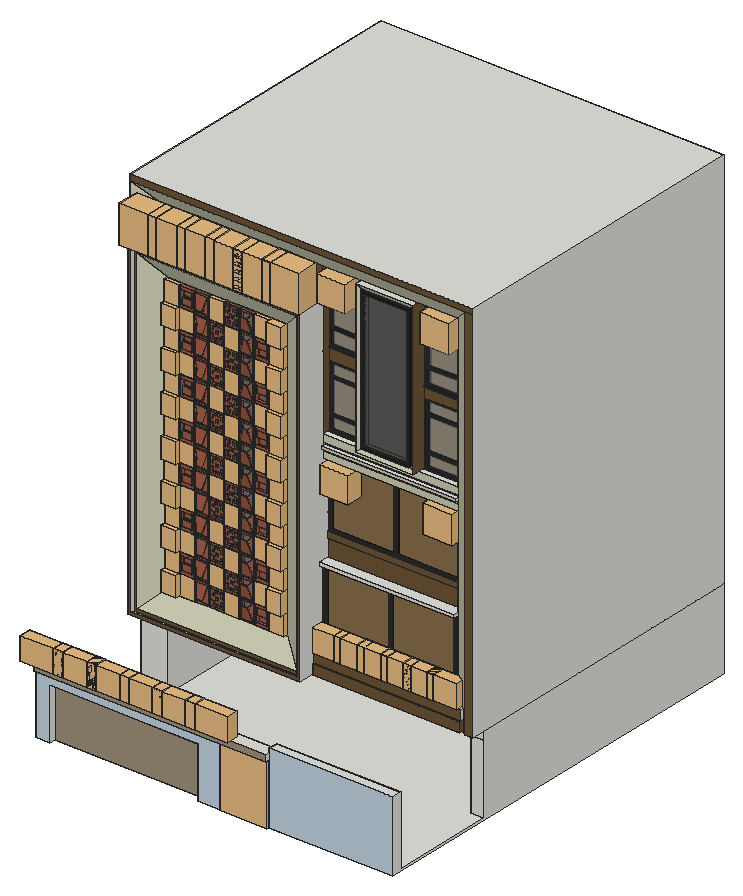
# SketchUp Ruby script. Lengths in inches.
U = 1.inch
M = Sketchup.active_model
def pt(a) = Geom::Point3d.new(a.map { |v| v * U })
def face(e, loops, mat)
  f = e.add_face(loops[0].map { |a| pt(a) })
  loops[1..].each { |l| e.add_face(l.map { |a| pt(a) }).erase! }
  f.material = f.back_material = mat if mat
  f
end
# faces: each face lists its corners as indices into pts; further lists are holes
def faces(e, pts, list, mat = nil) = list.each { |f| face(e, (f[0].is_a?(Array) ? f : [f]).map { |l| l.map { |i| pts[i] } }, mat) }
# xy, xz, yz: faces in a plane at the given z, y or x. An outline is a flat list of corners, or four numbers for a rectangle; further outlines are holes
def ring(l) = l.size == 4 ? [[l[0], l[1]], [l[2], l[1]], [l[2], l[3]], [l[0], l[3]]] : l.each_slice(2).to_a
def flat(e, list, mat, &to3) = list.each { |f| face(e, (f[0].is_a?(Array) ? f : [f]).map { |l| ring(l).map { |u, v| to3.(u, v) } }, mat) }
def xy(e, z, list, mat = nil) = flat(e, list, mat) { |x, y| [x, y, z] }
def xz(e, y, list, mat = nil) = flat(e, list, mat) { |x, z| [x, y, z] }
def yz(e, x, list, mat = nil) = flat(e, list, mat) { |y, z| [x, y, z] }
def lines(e, pts, list) = list.each { |a, b| e.add_line(pt(pts[a]), pt(pts[b])) }
# prism: a flat outline (further loops are holes) pulled along v
def prism(e, loops, v, mat = nil)
  f = face(e, loops, mat); d = Geom::Vector3d.new(v.map { |x| x * U })
  f.pushpull(f.normal.samedirection?(d) ? d.length : -d.length)
end
def box(e, o, s, mat = nil) = prism(e, [[o, [o[0] + s[0], o[1], o[2]], [o[0] + s[0], o[1] + s[1], o[2]], [o[0], o[1] + s[1], o[2]]]], [0, 0, s[2]], mat)
def at(x, y, z, deg = 0) = Geom::Transformation.translation(pt([x, y, z])) * Geom::Transformation.rotation(ORIGIN, Z_AXIS, deg.degrees)
def axes(o, x, y, z) = Geom::Transformation.new([*x, 0, *y, 0, *z, 0, *pt(o).to_a, 1])
def part(name) = M.definitions.add(name)
# library, detail: a bought-in or finely detailed component or shape, given as its bounding box
def library(name, o, s) = part(name).tap { |d| box(d.entities, o, s) }
def detail(e, o, s) = box(e.add_group.entities, o, s)
def put(e, d, t, mat = nil) = e.add_instance(d, t).tap { |i| i.material = mat if mat }
def group(e, t, mat = nil) = e.add_group.tap { |g| g.transformation = t; g.material = mat if mat }.entities
root = M.entities
M.materials.add("Concrete block").color = [182, 184, 178]
M.materials.add("Generic").color = [208, 207, 183]
M.materials.add("Glass_Tinted_Gray").color = [0, 0, 0]
M.materials["Glass_Tinted_Gray"].alpha = 0.125
M.materials.add("Sandstone 150cm").color = [161, 146, 124]
M.materials.add("Walnut Highgloss 300cm").color = [111, 85, 55]
M.materials.add("[0128_White]").color = [255, 255, 255]
M.materials.add("[0135_DarkGray]").color = [81, 81, 81]
M.materials.add("[Color C07]1").color = [160, 91, 69]
M.materials.add("[Color M01]").color = [226, 226, 226]
M.materials.add("[Color M07]").color = [114, 114, 114]
M.materials.add("[Color M08]").color = [30, 30, 30]
M.materials.add("[Granite Dark Gray]").color = [69, 68, 68]
M.materials.add("[Mirror 02]").color = [229, 229, 229]
M.materials.add("[Terrazzo Light Blue]").color = [196, 214, 227]
M.materials.add("[Translucent Glass Gray]").color = [51, 51, 51]
M.materials["[Translucent Glass Gray]"].alpha = 0.78
M.materials.add("[Translucent Glass Gray]2").color = [128, 128, 128]
M.materials["[Translucent Glass Gray]2"].alpha = 0.5
c1 = library("Paired curtain panels",[0.83,0,0],[155.09,8.12,139.81])
c2 = part("PENTEK_RP Fineline 50S_Sliding_DoorCase_E1")
box(c2.entities,[0,0,0],[1.51,3.66,99.27],"[0135_DarkGray]")
c3 = part("PENTEK_RP Fineline 50S_SlidingDooe_Case_E2")
box(c3.entities,[0,0,0],[96.25,3.66,1.51],"[0135_DarkGray]")
c4 = part("pentek_RP Fineline 50S_SlidingDoor_Case")
put(c4.entities,c2,at(97.76,0,0))
put(c4.entities,c3,at(1.51,0,0))
put(c4.entities,c2,at(0,0,0))
put(c4.entities,c3,at(1.51,0,97.76))
c5 = part("PENTEK_RP Fineline 50S_SlidingDoor_GlazingBead_2")
box(c5.entities,[0,0,0],[0.56,0.59,94.39],"[0135_DarkGray]")
c6 = part("PENTEK_RP Fineline 50S_SlidingDoor_Glass")
box(c6.entities,[0,0,0],[46.58,0.16,94.39],"Glass_Tinted_Gray")
c7 = part("PENTEK_RP Fineline 50S_SlidingDoor_GlazingBead")
box(c7.entities,[0,0,0],[45.47,0.59,0.56],"[0135_DarkGray]")
c8 = part("PENTEK_RP Fineline 50S_SlidingDoor_Leaf_E1")
xy(c8.entities,0,[[0,0,0.93,1.97],[0.93,1.57,1.49,1.97]],"[0135_DarkGray]")
xy(c8.entities,96.25,[[0,0,0.93,0,0.93,1.57,1.49,1.57,1.49,1.97,0,1.97]],"[0135_DarkGray]")
xz(c8.entities,0,[[0,0,0.93,96.25]],"[0135_DarkGray]")
xz(c8.entities,1.57,[[0.93,0,1.49,95.32],[0.93,95.32,1.49,96.25]],"[0135_DarkGray]")
xz(c8.entities,1.97,[[0,0,1.49,96.25]],"[0135_DarkGray]")
yz(c8.entities,0,[[0,0,1.97,96.25]],"[0135_DarkGray]")
yz(c8.entities,0.93,[[0,0,1.57,0.93],[0,0.93,1.57,95.32],[0,95.32,1.57,96.25]],"[0135_DarkGray]")
yz(c8.entities,1.49,[[1.57,0,1.97,95.32],[1.57,95.32,1.97,96.25]],"[0135_DarkGray]")
c9 = part("PENTEK_RP Fineline 50S_SlidingDoor_Leaf_E2")
xy(c9.entities,0,[[0,0,0,1.57,0.56,1.57,0.56,1.97,46.02,1.97,46.02,1.57,46.58,1.57,46.58,0]],"[0135_DarkGray]")
xy(c9.entities,0.93,[[0,0,46.58,1.57]],"[0135_DarkGray]")
xy(c9.entities,1.49,[[0.56,1.57,46.02,1.97]],"[0135_DarkGray]")
xz(c9.entities,0,[[0,0,46.58,0.93]],"[0135_DarkGray]")
xz(c9.entities,1.57,[[0,0,0.56,0.93],[46.02,0,46.58,0.93],[0.56,0.93,46.02,1.49]],"[0135_DarkGray]")
xz(c9.entities,1.97,[[0.56,0,46.02,1.49]],"[0135_DarkGray]")
yz(c9.entities,0,[[0,0,1.57,0.93]],"[0135_DarkGray]")
yz(c9.entities,0.56,[[1.57,0,1.97,0.93],[1.57,0.93,1.97,1.49]],"[0135_DarkGray]")
yz(c9.entities,46.02,[[1.57,0,1.97,0.93],[1.57,0.93,1.97,1.49]],"[0135_DarkGray]")
yz(c9.entities,46.58,[[0,0,1.57,0.93]],"[0135_DarkGray]")
c10 = part("PENTEK_RP Fineline S_SlidingDoor_Leaf1")
put(c10.entities,c5,at(0.93,0,0.93))
put(c10.entities,c5,at(46.96,0,0.93))
put(c10.entities,c6,at(1.49,1.42,0.93))
put(c10.entities,c7,at(1.49,0,0.93))
put(c10.entities,c6,at(1.49,0.59,0.93),"[Terrazzo Light Blue]")
put(c10.entities,c8,at(0,0,0))
put(c10.entities,c8,axes([48.44,0,0],[-1,0,0],[0,1,0],[0,0,1]))
put(c10.entities,c9,axes([0.93,0,96.25],[1,0,0],[0,1,0],[0,0,-1]))
put(c10.entities,c9,at(0.93,0,0))
put(c10.entities,c7,at(1.49,0,94.77))
c11 = part("PENTEK_RP Fineline 50S_SlidingDoor_Leaf2")
put(c11.entities,c6,at(1.49,1.42,0.93))
put(c11.entities,c7,at(1.49,0,94.77))
put(c11.entities,c5,at(46.96,0,0.93))
put(c11.entities,c6,at(1.49,0.59,0.93),"[Mirror 02]")
put(c11.entities,c5,at(0.93,0,0.93))
put(c11.entities,c8,at(0,0,0))
put(c11.entities,c8,axes([48.44,0,0],[-1,0,0],[0,1,0],[0,0,1]))
put(c11.entities,c7,at(1.49,0,0.93))
put(c11.entities,c9,axes([0.93,0,96.25],[1,0,0],[0,1,0],[0,0,-1]))
put(c11.entities,c9,at(0.93,0,0))
c12 = part("PENTEK - Slimmest Steel Sliding Door / Window\#1")
put(c12.entities,c4,at(0,-1.88,-0.09))
put(c12.entities,c10,at(1.51,-2.27,1.42))
put(c12.entities,c11,at(49.32,-0.3,1.42))
c13 = part("Agrupar\#57")
prism(c13.entities,[[[1.18,24.41,51.97],[1.18,0,51.97],[1.18,0,0],[1.18,24.41,0]],[[1.18,1.57,50.39],[1.18,22.83,50.39],[1.18,22.83,1.57],[1.18,1.57,1.57]]],[-1.18,0,0])
c14 = part("Agrupar\#59")
box(c14.entities,[0,0,0],[0.24,21.26,16.54])
c15 = part("Agrupar\#58")
prism(c15.entities,[[[0,0,0],[0,0,19.69],[0,24.41,19.69],[0,24.41,0]],[[0,1.57,1.57],[0,22.83,1.57],[0,22.83,18.11],[0,1.57,18.11]]],[1.18,0,0])
c16 = part("Agrupar\#56")
box(c16.entities,[0,0,0],[4.72,24.41,1.57])
c17 = part("Agrupar\#55")
prism(c17.entities,[[[0,0,0],[0,0,97.64],[0,27.56,97.64],[0,27.56,0]],[[0,25.98,1.57],[0,25.98,96.0625],[0,1.57,96.0625],[0,1.57,1.57]]],[4.72,0,0])
c18 = part("Agrupar\#60")
box(c18.entities,[0,0,0],[0.24,21.26,48.82])
c19 = part("Janela Maxim ar")
put(c19.entities,c13,at(1.77,1.57,22.83))
put(c19.entities,c14,at(2.36,3.15,77.95),"[Translucent Glass Gray]2")
put(c19.entities,c15,at(1.77,1.57,1.57))
put(c19.entities,c16,at(0,1.57,74.8))
put(c19.entities,c16,at(0,1.57,21.26))
put(c19.entities,c15,at(1.77,1.57,76.38))
put(c19.entities,c17,at(0,0,0))
put(c19.entities,c14,at(2.36,3.15,3.15),"[Translucent Glass Gray]2")
put(c19.entities,c18,at(2.36,3.15,24.41),"[Translucent Glass Gray]2")
c20 = part("Agrupar\#54")
box(c20.entities,[0,0,0],[7.09,27.56,0.79])
c21 = part("JA-70x250")
put(c21.entities,c19,at(2.36,0,0.79),"[Color M08]")
put(c21.entities,c20,at(0,0,0),"[Granite Dark Gray]")
c22 = library("170_fin_black (1)",[-4.89,-2.76,-3.35],[51.16,5.67,71.46])
c23 = library("Plante \#58",[-0.43,-1.58,0],[20.84,18.06,17.59])
c24 = part("Group\#116")
box(c24.entities,[0,0,0],[5.51,2.76,0.51])
c25 = part("Decorative screen block \#3")
g1 = group(c25.entities,at(0,0,0))
xy(g1,0,[[[0.2,0.2,7.68,7.68],[1.18,1.18,6.69,6.69]]])
xy(g1,0.2,[[[0,0,7.875,7.875],[0.2,0.2,7.68,7.68]]])
xy(g1,3.74,[[[0,0,7.875,7.875],[0.2,0.2,7.68,7.68]]])
xy(g1,3.9375,[[[0.2,0.2,7.68,7.68],[1.18,1.18,6.69,6.69]]])
xz(g1,0,[[0,0.2,7.875,3.74]])
xz(g1,0.2,[[0.2,0,7.68,0.2],[0.2,3.74,7.68,3.9375]])
xz(g1,1.18,[[1.18,0,6.69,3.9375]])
xz(g1,6.69,[[1.18,0,6.69,3.9375]])
xz(g1,7.68,[[0.2,0,7.68,0.2],[0.2,3.74,7.68,3.9375]])
xz(g1,7.875,[[0,0.2,7.875,3.74]])
yz(g1,0,[[0,0.2,7.875,3.74]])
yz(g1,0.2,[[0.2,0,7.68,0.2],[0.2,3.74,7.68,3.9375]])
yz(g1,1.18,[[1.18,0,6.69,3.9375]])
yz(g1,6.69,[[1.18,0,6.69,3.9375]])
yz(g1,7.68,[[0.2,0,7.68,0.2],[0.2,3.74,7.68,3.9375]])
yz(g1,7.875,[[0,0.2,7.875,3.74]])
put(c25.entities,c24,at(1.18,1.18,2.83))
put(c25.entities,c24,at(1.18,3.9375,0.59))
c26 = part("Component\#2")
xy(c26.entities,0,[[[0,0,5.91,5.91],[0.39,0.39,5.51,5.51]]])
xy(c26.entities,2.36,[[[0,0,5.91,5.91],[0.39,0.39,5.51,5.51]],[5.43,5.16,5.51,5.17,5.51,5.51]])
xz(c26.entities,0,[[0,0,5.91,2.36]])
xz(c26.entities,0.39,[[0.39,0,5.51,2.36]])
xz(c26.entities,5.51,[[0.39,0,5.51,2.36]])
xz(c26.entities,5.91,[[0,0,5.91,2.36]])
yz(c26.entities,0,[[0,0,5.91,2.36]])
yz(c26.entities,0.39,[[0.39,0,5.51,0,5.51,2.36,5.23,2.21,0.67,2.21,0.39,2.36],[0.67,2.21,5.23,2.21,5.51,2.36,0.39,2.36]])
yz(c26.entities,4.33,[[1.78,4.3,1.5,4.45,4.41,4.45,4.13,4.3]])
yz(c26.entities,5.51,[[0.39,0,5.17,2.36],[5.17,0,5.51,2.36]])
yz(c26.entities,5.91,[[0,0,5.91,2.36]])
p = [[0.39,0.39,2.36],[4.33,1.5,4.45],[4.33,1.78,4.3],[0.39,0.67,2.21],[5.51,0.39,2.36],[5.51,0.67,2.21],
  [5.43,0.75,2.36],[4.41,1.7,4.16],[0.39,5.23,2.21],[4.33,4.13,4.3],[5.51,5.23,2.21],[5.43,5.16,2.36],
  [4.33,4.41,4.45],[0.39,5.51,2.36],[5.51,5.51,2.36],[5.36,0.89,2.64],[4.49,1.7,4.18],[4.49,4.2,4.18],
  [5.36,5.02,2.64],[5.51,5.17,2.36],[5.51,0.74,2.36]]
faces(c26.entities,p,[[0,1,2,3],[4,0,3,5],[1,4,5,6,7,2],[5,3,2,7,6],[8,10,11,9],[12,13,8,9],[13,14,10,8],[0,4,1],
  [1,12,13,0],[15,16,17,18,19,14,12,1,4,20],[7,16,15,20,6],[9,11,14,12],[14,13,12]])
faces(c26.entities,p,[[8,3,2,9]],"[0128_White]")
c27 = part("Decorative screen block \#2")
xy(c27.entities,0,[[[0.2,0.2,7.68,7.68],[0.82,4.56,2.07,4.56,2.07,5.81,3.3125,5.81,3.3125,7.05,0.82,7.05],[0.82,0.82,3.3125,0.82,3.3125,2.07,2.07,2.07,2.07,3.3125,0.82,3.3125],[4.56,0.82,7.05,0.82,7.05,3.3125,5.81,3.3125,5.81,2.07,4.56,2.07],[5.81,4.56,7.05,4.56,7.05,7.05,4.56,7.05,4.56,5.81,5.81,5.81],[3.3125,3.3125,4.56,4.56]]])
xy(c27.entities,0.2,[[[0,0,7.875,7.875],[0.2,0.2,7.68,7.68]]])
xy(c27.entities,3.74,[[[0,0,7.875,7.875],[0.2,0.2,7.68,7.68]]])
xy(c27.entities,3.9375,[[[0.2,0.2,7.68,7.68],[0.82,0.82,0.82,3.3125,2.07,3.3125,2.07,2.07,3.3125,2.07,3.3125,0.82],[0.82,4.56,0.82,7.05,3.3125,7.05,3.3125,5.81,2.07,5.81,2.07,4.56],[4.56,0.82,4.56,2.07,5.81,2.07,5.81,3.3125,7.05,3.3125,7.05,0.82],[5.81,4.56,5.81,5.81,4.56,5.81,4.56,7.05,7.05,7.05,7.05,4.56],[3.3125,3.3125,4.56,4.56]]])
xz(c27.entities,0,[[0,0.2,7.875,3.74]])
xz(c27.entities,0.2,[[0.2,0,7.68,0.2],[0.2,3.74,7.68,3.9375]])
xz(c27.entities,0.82,[[0.82,0,3.3125,3.9375],[4.56,0,7.05,3.9375]])
xz(c27.entities,2.07,[[2.07,0,3.3125,3.9375],[4.56,0,5.81,3.9375]])
xz(c27.entities,3.3125,[[0.82,0,2.07,3.9375],[3.3125,0,4.56,3.9375],[5.81,0,7.05,3.9375]])
xz(c27.entities,4.56,[[0.82,0,2.07,3.9375],[3.3125,0,4.56,3.9375],[5.81,0,7.05,3.9375]])
xz(c27.entities,5.81,[[2.07,0,3.3125,3.9375],[4.56,0,5.81,3.9375]])
xz(c27.entities,7.05,[[0.82,0,3.3125,3.9375],[4.56,0,7.05,3.9375]])
xz(c27.entities,7.68,[[0.2,0,7.68,0.2],[0.2,3.74,7.68,3.9375]])
xz(c27.entities,7.875,[[0,0.2,7.875,3.74]])
yz(c27.entities,0,[[0,0.2,7.875,3.74]])
yz(c27.entities,0.2,[[0.2,0,7.68,0.2],[0.2,3.74,7.68,3.9375]])
yz(c27.entities,0.82,[[0.82,0,3.3125,3.9375],[4.56,0,7.05,3.9375]])
yz(c27.entities,2.07,[[2.07,0,3.3125,3.9375],[4.56,0,5.81,3.9375]])
yz(c27.entities,3.3125,[[0.82,0,2.07,3.9375],[3.3125,0,4.56,3.9375],[5.81,0,7.05,3.9375]])
yz(c27.entities,4.56,[[0.82,0,2.07,3.9375],[3.3125,0,4.56,3.9375],[5.81,0,7.05,3.9375]])
yz(c27.entities,5.81,[[2.07,0,3.3125,3.9375],[4.56,0,5.81,3.9375]])
yz(c27.entities,7.05,[[0.82,0,3.3125,3.9375],[4.56,0,7.05,3.9375]])
yz(c27.entities,7.68,[[0.2,0,7.68,0.2],[0.2,3.74,7.68,3.9375]])
yz(c27.entities,7.875,[[0,0.2,7.875,3.74]])
c28 = library("Circular opening block",[0,0,-3.9375],[7.875,7.875,7.875])
c29 = library("Decorative screen block \#1",[0,0,0],[7.875,7.875,3.9375])
c30 = library("Decorative screen block",[0,0,0],[7.875,7.875,3.9375])
c31 = library("Group\#2",[0,0,0],[7.875,2.95,7.875])
c32 = library("Group\#18",[0,0,0],[56.8,25.91,35.15])
c33 = part("Group\#19")
put(c33.entities,c32,at(0,0,0))
put(c33.entities,c32,at(88.8,0,0))
put(c33.entities,c32,at(133.08,0,0))
put(c33.entities,c32,at(176.53,0,0))
put(c33.entities,c32,at(44.08,0,0))
put(c33.entities,c32,at(220.58,0,0))
xy(root,-176,[[0,5.8125,0,29.26,29.875,29.26,29.875,909.1875,776.9375,909.1875,776.9375,8.9375,506.3125,8.9375,506.3125,29.26,402.62,29.26,402.62,5.8125,353.78,5.8125,353.78,20,29.875,20,29.875,5.8125]])
xy(root,-169.65,[[29.875,29.26,776.9375,29.26,776.9375,254.75,748.71,254.75,748.71,599.49,87.84,599.49,87.84,254.75,29.875,254.75]])
xy(root,-63.625,[[29.875,5.8125,353.78,20]],"[Color M01]")
xy(root,-42.84,[[0,0,402.62,5.8125],[402.62,0,506.3125,29.26]])
xy(root,-30.4,[[0,0,506.3125,29.26]])
xy(root,-20.71,[[506.3125,8.9375,776.9375,29.26]])
xy(root,-18.41,[[87.84,254.75,748.25,599.49]])
xy(root,0,[[51.21,193.0625,51.21,241.21,69.25,254.75,426.53,254.75,426.53,193.0625],[29.875,225.1875,29.875,254.75,51.21,254.75,51.21,241.21],[428.22,225.1875,428.22,254.75,720.57,254.75,748.19,234.01,748.19,225.1875],[759.9375,225.1875,748.19,234.01,748.19,254.75,776.9375,254.75,776.9375,225.1875],[748.19,234.01,720.57,254.75,748.19,254.75],
  [51.21,241.21,51.21,254.75,69.25,254.75]])
xy(root,6.33,[[57.32,193.0625,418.71,200.1875]])
xy(root,21.47,[[428.22,225.1875,748.19,227.875],[417.03,227.875,428.22,254.75]])
xy(root,42.94,[[417.03,227.875,748.19,227.875,748.19,254.75,720.57,254.75,720.57,396.1875,426.53,396.1875,426.53,254.75,417.03,254.75],[69.25,254.75,337.16,340]])
xy(root,205.02,[[426.53,244,720.57,396.1875]])
xy(root,211.66,[[426.53,244,720.57,268.6875]])
xy(root,250.25,[[426.53,265.8125,720.57,268.6875]],"Walnut Highgloss 300cm")
xy(root,262.7,[[426.53,265.8125,720.57,396.1875]])
xy(root,409.9,[[426.53,254.75,720.57,396.1875]])
xy(root,423.97,[[426.53,254.75,720.57,260.875]])
xy(root,429.89,[[426.53,249.6875,720.57,260.875]])
xy(root,435.28,[[426.53,249.6875,720.57,260.875]])
xy(root,441.875,[[426.53,254.75,720.57,260.875]])
xy(root,456.91,[[509.22,240.4375,635.07,254.75],[426.53,254.75,509.22,301.0625],[635.07,254.75,720.57,328.8125]])
xy(root,472.53,[[524.84,246.3125,619.45,255.3125]])
xy(root,593.92,[[426.53,270.5,509.22,301.0625],[635.07,270.5,720.57,328.8125]],"Walnut Highgloss 300cm")
xy(root,621.56,[[426.53,270.5,720.57,270.5,720.57,332.375,635.07,332.375,635.07,280.1875,509.22,280.1875,509.22,359.25,426.53,359.25]])
xy(root,715.08,[[57.32,193.0625,418.71,200.1875]])
xy(root,723.83,[[51.21,193.0625,426.53,254.75]])
xy(root,770.64,[[524.84,246.3125,619.45,255.3125]])
xy(root,786.25,[[509.22,240.4375,635.07,254.75],[509.22,254.75,635.07,280.1875]])
xy(root,786.25,[[69.25,254.75,337.16,340],[426.53,254.75,509.22,359.25],[635.07,254.75,720.57,332.375]],"Walnut Highgloss 300cm")
xy(root,838.25,[[29.875,225.1875,776.9375,909.1875]])
xz(root,0,[[0,-42.84,506.3125,-30.4]],"Sandstone 150cm")
xz(root,5.8125,[[0,-176,29.875,-176,29.875,-63.625,353.78,-63.625,353.78,-176,402.62,-176,402.62,-42.84,0,-42.84]],"[Terrazzo Light Blue]")
xz(root,8.9375,[[506.3125,-176,776.9375,-20.71]],"[Terrazzo Light Blue]")
xz(root,20,[[29.875,-176,353.78,-63.625]],"Sandstone 150cm")
xz(root,29.26,[[0,-176,29.875,-149.09],[402.62,-176,506.3125,-169.65],[29.875,-169.65,29.875,-149.09,0,-149.09,0,-30.4,506.3125,-30.4,506.3125,-20.71,776.9375,-20.71,776.9375,-169.65,506.3125,-169.65,506.3125,-42.84,402.62,-42.84,402.62,-169.65]])
xz(root,193.0625,[[[51.21,0,426.53,723.83],[57.32,6.33,418.71,715.08]]],"Walnut Highgloss 300cm")
xz(root,200.1875,[[[57.32,6.33,418.71,715.08],[64.43,11.86,413.4,707.9375]]],"Walnut Highgloss 300cm")
xz(root,225.1875,[[428.22,0,748.19,21.47],[759.9375,0,776.9375,825.625],[29.875,825.625,776.9375,838.25]],"Walnut Highgloss 300cm")
xz(root,227.875,[[417.03,21.47,748.19,42.94]],"Walnut Highgloss 300cm")
xz(root,229.16,[[108.57,56.16,369.26,663.64]],"[Color M07]")
xz(root,244,[[426.53,205.02,720.57,211.66]])
xz(root,246.3125,[[[518.98,466.67,625.3125,776.5],[524.84,472.53,619.45,770.64]]])
xz(root,249.6875,[[426.53,429.89,720.57,435.28]],"Generic")
xz(root,254.75,[[29.875,-169.65,87.84,0],[748.71,-169.65,776.9375,-169.65,776.9375,-18.41,748.25,-18.41],[87.84,-18.41,748.25,-18.41,748.19,0,87.84,0],[748.25,-18.41,776.9375,-18.41,776.9375,0,748.19,0],[51.21,0,69.25,723.83],
  [69.25,0,426.53,0,426.53,21.47,417.03,21.47,417.03,42.94,69.25,42.94],[426.53,0,428.22,21.47],[720.57,0,748.19,21.47],[417.03,21.47,426.53,42.94],[720.57,21.47,748.19,42.94],
  [69.25,42.94,337.16,723.83]])
xz(root,254.75,[[426.53,409.9,720.57,423.97],[426.53,441.875,720.57,456.91]],"Generic")
xz(root,254.75,[[337.16,723.83,426.53,786.25]],"Walnut Highgloss 300cm")
xz(root,255.3125,[[524.84,472.53,619.45,770.64]])
xz(root,260.875,[[426.53,423.97,720.57,429.89],[426.53,435.28,720.57,441.875]],"Generic")
xz(root,265.8125,[[426.53,250.25,720.57,262.7]],"Walnut Highgloss 300cm")
xz(root,268.6875,[[426.53,211.66,720.57,250.25]],"Walnut Highgloss 300cm")
xz(root,270.5,[[426.53,593.92,509.22,621.56],[635.07,593.92,720.57,621.56]],"Walnut Highgloss 300cm")
xz(root,280.1875,[[509.22,593.92,635.07,621.56]])
xz(root,301.0625,[[426.53,456.91,509.22,593.92]])
xz(root,328.8125,[[635.07,456.91,720.57,593.92]])
xz(root,332.375,[[635.07,621.56,720.57,786.25]])
xz(root,340,[[69.25,42.94,337.16,786.25]],"Walnut Highgloss 300cm")
xz(root,359.25,[[426.53,621.56,509.22,786.25]])
xz(root,396.1875,[[426.53,42.94,720.57,205.02],[426.53,262.7,720.57,409.9]])
xz(root,599.49,[[87.84,-169.65,748.71,-169.65,748.25,-18.41,87.84,-18.41]])
xz(root,909.1875,[[29.875,-176,776.9375,838.25]])
yz(root,0,[[5.8125,-176,5.8125,-42.84,0,-42.84,0,-30.4,29.26,-30.4,29.26,-176]])
yz(root,29.875,[[29.26,-176,29.26,-169.65,254.75,-169.65,254.75,0,225.1875,0,225.1875,838.25,909.1875,838.25,909.1875,-176]])
yz(root,29.875,[[5.8125,-176,20,-63.625]],"[Color M01]")
yz(root,51.21,[[193.0625,0,254.75,723.83]])
yz(root,57.32,[[193.0625,6.33,200.1875,715.08]])
yz(root,69.25,[[254.75,42.94,340,786.25]],"Walnut Highgloss 300cm")
yz(root,87.84,[[254.75,-169.65,599.49,-18.41]])
yz(root,337.16,[[254.75,42.94,340,786.25]],"Walnut Highgloss 300cm")
yz(root,353.78,[[5.8125,-176,20,-63.625]],"[Color M01]")
yz(root,402.62,[[5.8125,-176,29.26,-42.84]])
yz(root,417.03,[[227.875,21.47,254.75,42.94]])
yz(root,418.71,[[193.0625,6.33,200.1875,715.08]])
yz(root,426.53,[[193.0625,0,254.75,0,254.75,205.02,244,205.02,244,211.66,268.6875,211.66,268.6875,250.25,265.8125,250.25,265.8125,262.7,396.1875,262.7,396.1875,409.9,254.75,409.9,254.75,429.89,249.6875,429.89,249.6875,435.28,254.75,435.28,254.75,723.83,193.0625,723.83],[254.75,42.94,396.1875,205.02],[244,205.02,254.75,211.66],[254.75,423.97,260.875,429.89],[249.6875,429.89,254.75,435.28],
  [254.75,435.28,260.875,441.875]])
yz(root,426.53,[[254.75,456.91,301.0625,456.91,301.0625,593.92,270.5,593.92,270.5,621.56,359.25,621.56,359.25,786.25,254.75,786.25]],"Walnut Highgloss 300cm")
yz(root,428.22,[[225.1875,0,254.75,21.47]])
yz(root,506.3125,[[8.9375,-176,29.26,-42.84],[0,-42.84,8.9375,-30.4],[8.9375,-30.4,29.26,-20.71]])
yz(root,509.22,[[270.5,456.91,301.0625,593.92],[280.1875,621.56,359.25,786.25]])
yz(root,509.22,[[240.4375,456.91,240.4375,786.25,280.1875,786.25,280.1875,593.92,270.5,593.92,270.5,456.91]],"Walnut Highgloss 300cm")
yz(root,524.84,[[246.3125,472.53,255.3125,770.64]])
yz(root,619.45,[[246.3125,472.53,255.3125,770.64]])
yz(root,635.07,[[240.4375,456.91,328.8125,456.91,328.8125,593.92,280.1875,593.92,280.1875,621.56,332.375,621.56,332.375,786.25,240.4375,786.25]],"Walnut Highgloss 300cm")
yz(root,720.57,[[254.75,42.94,396.1875,205.02],[244,205.02,254.75,211.66],[254.75,211.66,254.75,262.7,265.8125,262.7,265.8125,250.25,268.6875,250.25,268.6875,211.66],[254.75,262.7,396.1875,409.9],[249.6875,429.89,254.75,435.28]])
yz(root,720.57,[[254.75,423.97,260.875,429.89],[254.75,435.28,260.875,441.875]],"Generic")
yz(root,720.57,[[254.75,456.91,328.8125,593.92],[254.75,593.92,270.5,621.56],[254.75,621.56,332.375,786.25]],"Walnut Highgloss 300cm")
yz(root,748.19,[[227.875,21.47,254.75,42.94]])
yz(root,748.19,[[225.1875,0,254.75,21.47]],"Walnut Highgloss 300cm")
yz(root,776.9375,[[8.9375,-176,909.1875,-176,909.1875,0,254.75,0,254.75,-169.65,29.26,-169.65,29.26,-20.71,8.9375,-20.71],[225.1875,0,909.1875,838.25]])
p = [[748.71,254.75,-169.65],[748.25,254.75,-18.41],[748.25,599.49,-18.41],[748.71,599.49,-169.65],[29.875,225.1875,825.625],[29.875,225.1875,0],
  [51.21,241.21,0],[69.25,254.75,0],[69.25,254.75,42.94],[69.25,254.75,723.83],[69.25,254.75,786.25],[759.9375,225.1875,0],
  [759.9375,225.1875,825.625],[720.57,254.75,786.25],[720.57,254.75,621.56],[720.57,254.75,593.92],[720.57,254.75,456.91],[720.57,254.75,441.875],
  [720.57,254.75,435.28],[720.57,254.75,429.89],[720.57,254.75,423.97],[720.57,254.75,409.9],[720.57,254.75,262.7],[720.57,254.75,211.66],
  [720.57,254.75,205.02],[720.57,254.75,42.94],[720.57,254.75,21.47],[720.57,254.75,0],[748.19,234.01,0],[369.26,229.16,56.16],
  [108.57,229.16,56.16],[64.43,200.1875,11.86],[413.4,200.1875,11.86],[64.43,200.1875,707.9375],[108.57,229.16,663.64],[369.26,229.16,663.64],
  [413.4,200.1875,707.9375],[625.3125,246.3125,466.67],[518.98,246.3125,466.67],[509.22,240.4375,456.91],[635.07,240.4375,456.91],[509.22,240.4375,786.25],
  [518.98,246.3125,776.5],[625.3125,246.3125,776.5],[635.07,240.4375,786.25],[337.16,254.75,786.25],[417.84,254.75,786.25],[426.53,254.75,786.25],
  [509.22,254.75,786.25],[635.07,254.75,786.25]]
faces(root,p,[[0,1,2,3]])
faces(root,p,[[4,5,6,7,8,9,10],[11,12,13,14,15,16,17,18,19,20,21,22,23,24,25,26,27,28],[29,30,31,32],[33,31,30,34],[35,29,32,36],[37,38,39,40],[41,39,38,42],[43,37,40,44],
  [36,33,34,35],[44,41,42,43],[13,12,4,10,45,46,47,48,49]],"Generic")
put(root,c1,axes([424.96,261.8125,42.94],[1.89585,0,0],[0,1.5,0],[0,0,1.15927]))
put(root,c1,axes([424.96,280.17,262.7],[1.89585,0,0],[0,1.5,0],[0,0,1.05288]))
put(root,c1,axes([424.96,280.17,456.91],[1.89585,0,0],[0,1.5,0],[0,0,0.98]))
put(root,c1,axes([423.34,280.0625,621.56],[1.89585,0,0],[0,1.5,0],[0,0,1.17802]))
put(root,c12,axes([426.53,271.21,262.74],[2.96196,0,0],[0,1,0],[0,0,1.48371]))
put(root,c12,axes([426.53,256.63,43.09],[2.96196,0,0],[0,1,0],[0,0,1.63263]))
put(root,c21,axes([509.22,268.14,620.77],[0,1,0],[-3.00073,0,0],[0,0,1.6813]))
put(root,c21,axes([723.17,263.41,620.77],[0,1,0],[-3.00073,0,0],[0,0,1.6813]))
put(root,c21,axes([509.22,268.14,456.91],[0,1,0],[-3.00073,0,0],[0,0,1.39203]))
put(root,c21,axes([720.57,268.14,456.91],[0,1,0],[-3.10233,0,0],[0,0,1.39203]))
put(root,c22,axes([412.2,7.03,-169.76],[2,0,0],[0,1,0],[0,0,1.86352]))
put(root,c23,axes([436.82,237.1875,353.02],[2.93576,0,0],[0,1.96291,0],[0,0,3.23441]))
put(root,c23,axes([657.58,242.3,348.3125],[3.08632,0,0],[0,1.65258,0],[0,0,3.50172]))
put(root,c23,axes([657.58,234.64,724.67],[3.08632,0,0],[0,1.65258,0],[0,0,3.50172]))
put(root,c23,axes([436.82,229.53,729.37],[2.93576,0,0],[0,1.96291,0],[0,0,3.23441]))
g2 = group(root,at(108.57,211.46,56.16))
put(g2,c25,axes([228.03,8.95,0],[-4.07199,0,0],[0,0,5.51066],[0,2.2733,0]),"[Color C07]1")
put(g2,c26,axes([65.32,17.45,43.39],[0,0,-7.34755],[5.53067,0,0],[0,-3.43029,0]),"[Color C07]1")
put(g2,c27,axes([130.65,9.4,0],[-4.148,0,0],[0,0,5.51066],[0,2.14827,0]),"[Color C07]1")
put(g2,c28,axes([32.36,8.95,0],[-4.11028,0,0],[0,0,5.51066],[0,2.2733,0]),"[Color C07]1")
put(g2,c29,axes([163.21,8.95,0],[-4.13596,0,0],[0,0,5.51066],[0,2.2733,0]),"[Color C07]1")
put(g2,c30,axes([65.32,9.35,0],[-4.18948,0,0],[0,0,5.51066],[0,2.05817,0]),"[Color C07]1")
put(g2,c26,axes([195.97,17.45,0],[0,0,7.34755],[-5.53067,0,0],[0,-3.401,0]),"[Color C07]1")
put(g2,c31,axes([260.69,9,43.39],[-4.148,0,0],[0,2.86238,0],[0,0,-5.51066]),"[Color C07]1")
g3 = group(root,at(108.57,211.46,99.56))
put(g3,c25,axes([32.66,8.95,43.39],[4.07199,0,0],[0,0,-5.51066],[0,2.2733,0]),"[Color C07]1")
put(g3,c26,axes([64.72,17.45,43.39],[0,0,-7.34755],[5.53067,0,0],[0,-3.401,0]),"[Color C07]1")
put(g3,c29,axes([97.48,8.95,43.39],[4.13596,0,0],[0,0,-5.51066],[0,2.2733,0]),"[Color C07]1")
put(g3,c28,axes([228.33,8.95,43.39],[4.11028,0,0],[0,0,-5.51066],[0,2.2733,0]),"Concrete block")
put(g3,c26,axes([195.37,17.45,0],[0,0,7.34755],[-5.53067,0,0],[0,-3.43029,0]),"[Color C07]1")
put(g3,c27,axes([130.05,9.4,43.39],[4.148,0,0],[0,0,-5.51066],[0,2.14827,0]),"[Color C07]1")
put(g3,c30,axes([195.37,9.35,43.39],[4.18948,0,0],[0,0,-5.51066],[0,2.05817,0]),"[Color C07]1")
put(g3,c31,axes([0,9,0],[4.148,0,0],[0,2.86238,0],[0,0,5.51066]),"[Color C07]1")
g4 = group(root,at(108.57,211.06,576.86))
put(g4,c25,axes([228.03,8.95,0],[-4.07199,0,0],[0,0,5.51066],[0,2.2733,0]),"[Color C07]1")
put(g4,c26,axes([65.32,17.45,43.39],[0,0,-7.34755],[5.53067,0,0],[0,-3.43029,0]),"[Color C07]1")
put(g4,c27,axes([130.65,9.4,0],[-4.148,0,0],[0,0,5.51066],[0,2.14827,0]),"[Color C07]1")
put(g4,c28,axes([32.36,8.95,0],[-4.11028,0,0],[0,0,5.51066],[0,2.2733,0]),"[Color C07]1")
put(g4,c29,axes([163.21,8.95,0],[-4.13596,0,0],[0,0,5.51066],[0,2.2733,0]),"[Color C07]1")
put(g4,c30,axes([65.32,9.35,0],[-4.18948,0,0],[0,0,5.51066],[0,2.05817,0]),"[Color C07]1")
put(g4,c26,axes([195.97,17.45,0],[0,0,7.34755],[-5.53067,0,0],[0,-3.401,0]),"[Color C07]1")
put(g4,c31,axes([260.69,9,43.39],[-4.148,0,0],[0,2.86238,0],[0,0,-5.51066]))
g5 = group(root,at(108.57,210.66,533.47))
put(g5,c25,axes([32.66,8.95,43.39],[4.07199,0,0],[0,0,-5.51066],[0,2.2733,0]),"[Color C07]1")
put(g5,c26,axes([64.72,17.45,43.39],[0,0,-7.34755],[5.53067,0,0],[0,-3.401,0]),"[Color C07]1")
put(g5,c29,axes([97.48,8.95,43.39],[4.13596,0,0],[0,0,-5.51066],[0,2.2733,0]),"[Color C07]1")
put(g5,c28,axes([228.33,8.95,43.39],[4.11028,0,0],[0,0,-5.51066],[0,2.2733,0]),"[Color C07]1")
put(g5,c26,axes([195.37,17.45,0],[0,0,7.34755],[-5.53067,0,0],[0,-3.43029,0]),"[Color C07]1")
put(g5,c27,axes([130.05,9.4,43.39],[4.148,0,0],[0,0,-5.51066],[0,2.14827,0]),"[Color C07]1")
put(g5,c30,axes([195.37,9.35,43.39],[4.18948,0,0],[0,0,-5.51066],[0,2.05817,0]),"[Color C07]1")
put(g5,c31,axes([0,9,0],[4.148,0,0],[0,2.86238,0],[0,0,5.51066]))
g6 = group(root,at(108.57,210.66,446.68))
put(g6,c25,axes([32.66,8.95,43.39],[4.07199,0,0],[0,0,-5.51066],[0,2.2733,0]),"[Color C07]1")
put(g6,c26,axes([64.72,17.45,43.39],[0,0,-7.34755],[5.53067,0,0],[0,-3.401,0]),"[Color C07]1")
put(g6,c29,axes([97.48,8.95,43.39],[4.13596,0,0],[0,0,-5.51066],[0,2.2733,0]),"[Color C07]1")
put(g6,c28,axes([228.33,8.95,43.39],[4.11028,0,0],[0,0,-5.51066],[0,2.2733,0]),"[Color C07]1")
put(g6,c26,axes([195.37,17.45,0],[0,0,7.34755],[-5.53067,0,0],[0,-3.43029,0]),"[Color C07]1")
put(g6,c27,axes([130.05,9.4,43.39],[4.148,0,0],[0,0,-5.51066],[0,2.14827,0]),"[Color C07]1")
put(g6,c30,axes([195.37,9.35,43.39],[4.18948,0,0],[0,0,-5.51066],[0,2.05817,0]),"[Color C07]1")
put(g6,c31,axes([0,9,0],[4.148,0,0],[0,2.86238,0],[0,0,5.51066]))
g7 = group(root,at(108.57,211.06,490.07))
put(g7,c25,axes([228.03,8.95,0],[-4.07199,0,0],[0,0,5.51066],[0,2.2733,0]),"[Color C07]1")
put(g7,c26,axes([65.32,17.45,43.39],[0,0,-7.34755],[5.53067,0,0],[0,-3.43029,0]),"[Color C07]1")
put(g7,c27,axes([130.65,9.4,0],[-4.148,0,0],[0,0,5.51066],[0,2.14827,0]),"[Color C07]1")
put(g7,c28,axes([32.36,8.95,0],[-4.11028,0,0],[0,0,5.51066],[0,2.2733,0]),"[Color C07]1")
put(g7,c29,axes([163.21,8.95,0],[-4.13596,0,0],[0,0,5.51066],[0,2.2733,0]),"[Color C07]1")
put(g7,c30,axes([65.32,9.35,0],[-4.18948,0,0],[0,0,5.51066],[0,2.05817,0]),"[Color C07]1")
put(g7,c26,axes([195.97,17.45,0],[0,0,7.34755],[-5.53067,0,0],[0,-3.401,0]),"[Color C07]1")
put(g7,c31,axes([260.69,9,43.39],[-4.148,0,0],[0,2.86238,0],[0,0,-5.51066]))
g8 = group(root,at(108.57,211.46,186.34))
put(g8,c25,axes([32.66,8.95,43.39],[4.07199,0,0],[0,0,-5.51066],[0,2.2733,0]),"[Color C07]1")
put(g8,c26,axes([64.72,17.45,43.39],[0,0,-7.34755],[5.53067,0,0],[0,-3.401,0]),"[Color C07]1")
put(g8,c29,axes([97.48,8.95,43.39],[4.13596,0,0],[0,0,-5.51066],[0,2.2733,0]),"[Color C07]1")
put(g8,c28,axes([228.33,8.95,43.39],[4.11028,0,0],[0,0,-5.51066],[0,2.2733,0]),"[Color C07]1")
put(g8,c26,axes([195.37,17.45,0],[0,0,7.34755],[-5.53067,0,0],[0,-3.43029,0]),"[Color C07]1")
put(g8,c27,axes([130.05,9.4,43.39],[4.148,0,0],[0,0,-5.51066],[0,2.14827,0]),"[Color C07]1")
put(g8,c30,axes([195.37,9.35,43.39],[4.18948,0,0],[0,0,-5.51066],[0,2.05817,0]),"[Color C07]1")
put(g8,c31,axes([0,9,0],[4.148,0,0],[0,2.86238,0],[0,0,5.51066]))
g9 = group(root,at(108.57,211.06,316.51))
put(g9,c25,axes([228.03,8.95,0],[-4.07199,0,0],[0,0,5.51066],[0,2.2733,0]),"[Color C07]1")
put(g9,c26,axes([65.32,17.45,43.39],[0,0,-7.34755],[5.53067,0,0],[0,-3.43029,0]),"[Color C07]1")
put(g9,c27,axes([130.65,9.4,0],[-4.148,0,0],[0,0,5.51066],[0,2.14827,0]),"[Color C07]1")
put(g9,c28,axes([32.36,8.95,0],[-4.11028,0,0],[0,0,5.51066],[0,2.2733,0]),"[Color C07]1")
put(g9,c29,axes([163.21,8.95,0],[-4.13596,0,0],[0,0,5.51066],[0,2.2733,0]),"[Color C07]1")
put(g9,c30,axes([65.32,9.35,0],[-4.18948,0,0],[0,0,5.51066],[0,2.05817,0]),"[Color C07]1")
put(g9,c26,axes([195.97,17.45,0],[0,0,7.34755],[-5.53067,0,0],[0,-3.401,0]),"[Color C07]1")
put(g9,c31,axes([260.69,9,43.39],[-4.148,0,0],[0,2.86238,0],[0,0,-5.51066]))
g10 = group(root,at(108.57,211.06,273.12))
put(g10,c25,axes([32.66,8.95,43.39],[4.07199,0,0],[0,0,-5.51066],[0,2.2733,0]),"[Color C07]1")
put(g10,c26,axes([64.72,17.45,43.39],[0,0,-7.34755],[5.53067,0,0],[0,-3.401,0]),"[Color C07]1")
put(g10,c29,axes([97.48,8.95,43.39],[4.13596,0,0],[0,0,-5.51066],[0,2.2733,0]),"[Color C07]1")
put(g10,c28,axes([228.33,8.95,43.39],[4.11028,0,0],[0,0,-5.51066],[0,2.2733,0]),"[Color C07]1")
put(g10,c26,axes([195.37,17.45,0],[0,0,7.34755],[-5.53067,0,0],[0,-3.43029,0]),"[Color C07]1")
put(g10,c27,axes([130.05,9.4,43.39],[4.148,0,0],[0,0,-5.51066],[0,2.14827,0]),"[Color C07]1")
put(g10,c30,axes([195.37,9.35,43.39],[4.18948,0,0],[0,0,-5.51066],[0,2.05817,0]),"[Color C07]1")
put(g10,c31,axes([0,9,0],[4.148,0,0],[0,2.86238,0],[0,0,5.51066]))
g11 = group(root,at(108.57,211.46,142.95))
put(g11,c25,axes([228.03,8.95,0],[-4.07199,0,0],[0,0,5.51066],[0,2.2733,0]),"[Color C07]1")
put(g11,c26,axes([65.32,17.45,43.39],[0,0,-7.34755],[5.53067,0,0],[0,-3.43029,0]),"[Color C07]1")
put(g11,c27,axes([130.65,9.4,0],[-4.148,0,0],[0,0,5.51066],[0,2.14827,0]),"[Color C07]1")
put(g11,c28,axes([32.36,8.95,0],[-4.11028,0,0],[0,0,5.51066],[0,2.2733,0]),"[Color C07]1")
put(g11,c29,axes([163.21,8.95,0],[-4.13596,0,0],[0,0,5.51066],[0,2.2733,0]),"[Color C07]1")
put(g11,c30,axes([65.32,9.35,0],[-4.18948,0,0],[0,0,5.51066],[0,2.05817,0]),"[Color C07]1")
put(g11,c26,axes([195.97,17.45,0],[0,0,7.34755],[-5.53067,0,0],[0,-3.401,0]),"[Color C07]1")
put(g11,c31,axes([260.69,9,43.39],[-4.148,0,0],[0,2.86238,0],[0,0,-5.51066]))
g12 = group(root,at(108.57,210.66,359.9))
put(g12,c25,axes([32.66,8.95,43.39],[4.07199,0,0],[0,0,-5.51066],[0,2.2733,0]),"[Color C07]1")
put(g12,c26,axes([64.72,17.45,43.39],[0,0,-7.34755],[5.53067,0,0],[0,-3.401,0]),"[Color C07]1")
put(g12,c29,axes([97.48,8.95,43.39],[4.13596,0,0],[0,0,-5.51066],[0,2.2733,0]),"[Color C07]1")
put(g12,c28,axes([228.33,8.95,43.39],[4.11028,0,0],[0,0,-5.51066],[0,2.2733,0]),"[Color C07]1")
put(g12,c26,axes([195.37,17.45,0],[0,0,7.34755],[-5.53067,0,0],[0,-3.43029,0]),"[Color C07]1")
put(g12,c27,axes([130.05,9.4,43.39],[4.148,0,0],[0,0,-5.51066],[0,2.14827,0]),"[Color C07]1")
put(g12,c30,axes([195.37,9.35,43.39],[4.18948,0,0],[0,0,-5.51066],[0,2.05817,0]),"[Color C07]1")
put(g12,c31,axes([0,9,0],[4.148,0,0],[0,2.86238,0],[0,0,5.51066]))
g13 = group(root,at(108.57,211.06,403.29))
put(g13,c25,axes([228.03,8.95,0],[-4.07199,0,0],[0,0,5.51066],[0,2.2733,0]),"[Color C07]1")
put(g13,c26,axes([65.32,17.45,43.39],[0,0,-7.34755],[5.53067,0,0],[0,-3.43029,0]),"[Color C07]1")
put(g13,c27,axes([130.65,9.4,0],[-4.148,0,0],[0,0,5.51066],[0,2.14827,0]),"[Color C07]1")
put(g13,c28,axes([32.36,8.95,0],[-4.11028,0,0],[0,0,5.51066],[0,2.2733,0]),"[Color C07]1")
put(g13,c29,axes([163.21,8.95,0],[-4.13596,0,0],[0,0,5.51066],[0,2.2733,0]),"[Color C07]1")
put(g13,c30,axes([65.32,9.35,0],[-4.18948,0,0],[0,0,5.51066],[0,2.05817,0]),"[Color C07]1")
put(g13,c26,axes([195.97,17.45,0],[0,0,7.34755],[-5.53067,0,0],[0,-3.401,0]),"[Color C07]1")
put(g13,c31,axes([260.69,9,43.39],[-4.148,0,0],[0,2.86238,0],[0,0,-5.51066]))
g14 = group(root,at(108.57,211.46,229.73))
put(g14,c25,axes([228.03,8.95,0],[-4.07199,0,0],[0,0,5.51066],[0,2.2733,0]),"[Color C07]1")
put(g14,c26,axes([65.32,17.45,43.39],[0,0,-7.34755],[5.53067,0,0],[0,-3.43029,0]),"[Color C07]1")
put(g14,c27,axes([130.65,9.4,0],[-4.148,0,0],[0,0,5.51066],[0,2.14827,0]),"[Color C07]1")
put(g14,c28,axes([32.36,8.95,0],[-4.11028,0,0],[0,0,5.51066],[0,2.2733,0]),"[Color C07]1")
put(g14,c29,axes([163.21,8.95,0],[-4.13596,0,0],[0,0,5.51066],[0,2.2733,0]),"[Color C07]1")
put(g14,c30,axes([65.32,9.35,0],[-4.18948,0,0],[0,0,5.51066],[0,2.05817,0]),"[Color C07]1")
put(g14,c26,axes([195.97,17.45,0],[0,0,7.34755],[-5.53067,0,0],[0,-3.401,0]),"[Color C07]1")
put(g14,c31,axes([260.69,9,43.39],[-4.148,0,0],[0,2.86238,0],[0,0,-5.51066]),"[Color C07]1")
g15 = group(root,at(108.57,210.66,620.25))
put(g15,c25,axes([32.66,8.95,43.39],[4.07199,0,0],[0,0,-5.51066],[0,2.2733,0]),"[Color C07]1")
put(g15,c26,axes([64.72,17.45,43.39],[0,0,-7.34755],[5.53067,0,0],[0,-3.401,0]),"[Color C07]1")
put(g15,c29,axes([97.48,8.95,43.39],[4.13596,0,0],[0,0,-5.51066],[0,2.2733,0]),"[Color C07]1")
put(g15,c28,axes([228.33,8.95,43.39],[4.11028,0,0],[0,0,-5.51066],[0,2.2733,0]),"[Color C07]1")
put(g15,c26,axes([195.37,17.45,0],[0,0,7.34755],[-5.53067,0,0],[0,-3.43029,0]),"[Color C07]1")
put(g15,c27,axes([130.05,9.4,43.39],[4.148,0,0],[0,0,-5.51066],[0,2.14827,0]),"[Color C07]1")
put(g15,c30,axes([195.37,9.35,43.39],[4.18948,0,0],[0,0,-5.51066],[0,2.05817,0]),"[Color C07]1")
put(g15,c31,axes([0,9,0],[4.148,0,0],[0,2.86238,0],[0,0,5.51066]))
g16 = group(root,at(518.98,242.0625,466.67))
xy(g16,0,[[0,0,106.33,4.25]],"[Color M08]")
xy(g16,5.86,[[5.86,0,100.47,2.125],[5.86,2.125,100.47,4.25]])
xy(g16,303.97,[[5.86,0,100.47,2.125],[5.86,2.125,100.47,4.25]],"[Color M08]")
xy(g16,309.83,[[0,0,106.33,4.25]],"[Color M08]")
xz(g16,0,[[[0,0,106.33,309.83],[5.86,5.86,100.47,303.97]]],"[Color M08]")
xz(g16,2.125,[[5.86,5.86,100.47,303.97]],"[Translucent Glass Gray]")
xz(g16,4.25,[[[0,0,106.33,309.83],[5.86,5.86,100.47,303.97]]],"[Color M08]")
yz(g16,0,[[0,0,4.25,309.83]])
yz(g16,5.86,[[0,5.86,2.125,303.97],[2.125,5.86,4.25,303.97]],"[Color M08]")
yz(g16,100.47,[[0,5.86,2.125,303.97],[2.125,5.86,4.25,303.97]])
yz(g16,106.33,[[0,0,4.25,309.83]],"[Color M08]")
put(root,c33,axes([423.35,224.39,42.82],[1.15,0,0],[0,1,0],[0,0,1.43]))
put(root,c33,axes([41.96,180.84,723.82],[1.40864,0,0],[0,1.87,0],[0,0,2.31]))
put(root,c33,axes([-24.46,-6.61,-30.5625],[1.633,0,0],[0,1,0],[0,0,1.43]))
